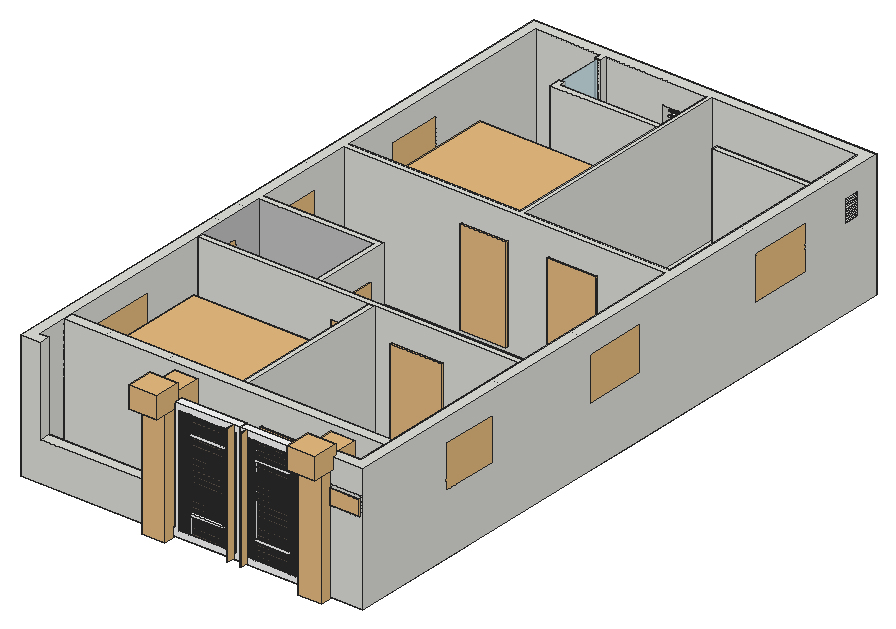
# SketchUp Ruby script. Lengths in inches.
U = 1.inch
M = Sketchup.active_model
def pt(a) = Geom::Point3d.new(a.map { |v| v * U })
def face(e, loops, mat)
  f = e.add_face(loops[0].map { |a| pt(a) })
  loops[1..].each { |l| e.add_face(l.map { |a| pt(a) }).erase! }
  f.material = f.back_material = mat if mat
  f
end
# faces: each face lists its corners as indices into pts; further lists are holes
def faces(e, pts, list, mat = nil) = list.each { |f| face(e, (f[0].is_a?(Array) ? f : [f]).map { |l| l.map { |i| pts[i] } }, mat) }
# xy, xz, yz: faces in a plane at the given z, y or x. An outline is a flat list of corners, or four numbers for a rectangle; further outlines are holes
def ring(l) = l.size == 4 ? [[l[0], l[1]], [l[2], l[1]], [l[2], l[3]], [l[0], l[3]]] : l.each_slice(2).to_a
def flat(e, list, mat, &to3) = list.each { |f| face(e, (f[0].is_a?(Array) ? f : [f]).map { |l| ring(l).map { |u, v| to3.(u, v) } }, mat) }
def xy(e, z, list, mat = nil) = flat(e, list, mat) { |x, y| [x, y, z] }
def xz(e, y, list, mat = nil) = flat(e, list, mat) { |x, z| [x, y, z] }
def yz(e, x, list, mat = nil) = flat(e, list, mat) { |y, z| [x, y, z] }
def lines(e, pts, list) = list.each { |a, b| e.add_line(pt(pts[a]), pt(pts[b])) }
# prism: a flat outline (further loops are holes) pulled along v
def prism(e, loops, v, mat = nil)
  f = face(e, loops, mat); d = Geom::Vector3d.new(v.map { |x| x * U })
  f.pushpull(f.normal.samedirection?(d) ? d.length : -d.length)
end
def box(e, o, s, mat = nil) = prism(e, [[o, [o[0] + s[0], o[1], o[2]], [o[0] + s[0], o[1] + s[1], o[2]], [o[0], o[1] + s[1], o[2]]]], [0, 0, s[2]], mat)
def at(x, y, z, deg = 0) = Geom::Transformation.translation(pt([x, y, z])) * Geom::Transformation.rotation(ORIGIN, Z_AXIS, deg.degrees)
def axes(o, x, y, z) = Geom::Transformation.new([*x, 0, *y, 0, *z, 0, *pt(o).to_a, 1])
def part(name) = M.definitions.add(name)
# library, detail: a bought-in or finely detailed component or shape, given as its bounding box
def library(name, o, s) = part(name).tap { |d| box(d.entities, o, s) }
def detail(e, o, s) = box(e.add_group.entities, o, s)
def put(e, d, t, mat = nil) = e.add_instance(d, t).tap { |i| i.material = mat if mat }
def group(e, t, mat = nil) = e.add_group.tap { |g| g.transformation = t; g.material = mat if mat }.entities
root = M.entities
M.materials.add("34af249def0fa13af67ab2bd33b938c5").color = [198, 197, 197]
M.materials.add("Steve_Edges").color = [0, 0, 0]
M.materials.add("[Color A04]").color = [128, 123, 118]
M.materials.add("[Color_000]").color = [255, 255, 255]
M.materials.add("[Color_C20]").color = [102, 91, 81]
M.materials.add("[Translucent Glass Safety]").color = [204, 235, 244]
M.materials["[Translucent Glass Safety]"].alpha = 0.5
c1 = library("A$C1EC128A1",[-3.37,-3.7,0],[6.74,7.4,0.01])
c2 = part("*U4")
p = [[-20,-17,0],[-20,23,0],[-18.25,23,0],[-18.25,-17,0],[20,-17,0],[19.92,-14.49,0],
  [19.68,-11.99,0],[19.29,-9.5,0],[18.74,-7.05,0],[18.04,-4.64,0],[17.19,-2.28,0],[16.19,0.03,0],
  [15.05,2.27,0],[13.77,4.43,0],[12.36,6.51,0],[10.82,8.5,0],[9.16,10.38,0],[7.38,12.16,0],
  [5.5,13.82,0],[3.51,15.36,0],[1.43,16.77,0],[-0.73,18.05,0],[-2.97,19.19,0],[-5.28,20.19,0],
  [-7.64,21.04,0],[-10.05,21.74,0],[-12.5,22.29,0],[-14.99,22.68,0],[-17.49,22.92,0],[-20,-23,0],
  [20,-23,0]]
lines(c2.entities,p,[[0,1],[1,2],[2,3],[3,0],[4,5],[5,6],[6,7],[7,8],[8,9],[9,10],[10,11],[11,12],
  [12,13],[13,14],[14,15],[15,16],[16,17],[17,18],[18,19],[19,20],[20,21],[21,22],[22,23],[23,24],
  [24,25],[25,26],[26,27],[27,28],[28,1],[0,29],[4,30]])
c3 = library("Кровать",[-17.4,-26.33,0],[117.11,127.46,87.48])
c4 = library("Plante \#58",[-0.43,-1.58,0],[20.84,18.06,17.59])
c5 = library("Wall mounted toilet",[0,0,0],[28.35,19.69,42.125])
c6 = library("RAGHU HOUSE NO:2",[0.29,0,0],[30,12.43,1])
c7 = part("Group20\#1")
xy(c7.entities,0,[[51,0,51,82.47,60,82.47,60,9,155.48,9,155.48,33.6875,161.25,33.6875,161.25,0],[309.375,0,309.375,9,330,9,330,96.75,339,96.75,339,0],[60,34,94.95,43],[94.95,34,147.28,37],[147.28,34,330,43],
  [94.95,39.54,147.28,43],[330,96.75,333.05,145.46],[333.05,96.75,335.78,145.46],[330,145.46,339,228.43],[60,175,330,180],
  [51,201.63,53.96,226.12],[56.65,201.63,60,226.12],[51,226.12,60,273.45],[332.92,228.43,335.82,280.48],[51,273.45,53.82,296.92],
  [330,407.14,332.19,455.17],[335.62,407.14,339,455.17],[51,416.55,51,540,146.27,540,146.27,531,119,531,119,525.5625,114,525.5625,114,531,60,531,60,416.55],[114,478,114,487.41,116.04,487.41,116.04,525.5625,116.5,525.5625,116.5,487.41,119,487.41,119,483,204,483,204,478],[250.49,478,330,483],
  [330,491.8,333.45,519.52],[333.45,491.8,336.34,519.52],[330,519.52,330,531,169.99,531,169.99,540,339,540,339,519.52]])
xy(c7.entities,4,[[226.66,34,272.82,43],[171.75,175,200.82,180],[223.46,175,266.65,180],[156,203.83,161,228.59],[158.97,329,197.75,334],
  [231.92,329,272.96,334]])
xy(c7.entities,33.15,[[67.875,0,161.25,0,161.25,33.6875,155.48,33.6875,155.48,9,67.875,9]])
xy(c7.entities,51,[[51,67.95,60,121.625],[330,87.84,339,136.4],[51,191.41,60,215.55],[330,239.56,339,290.25],[51,257.89,60,297.67],
  [51,379.57,60,425.91],[330,412.9375,339,464.66]])
xy(c7.entities,67.875,[[166.625,531,185.79,540]])
xy(c7.entities,68.5625,[[330,507.05,339,520.18]])
xy(c7.entities,84,[[226.66,34,272.82,43],[171.75,175,200.82,180],[223.46,175,266.65,180],[156,203.83,161,228.59],[158.97,329,197.75,334],
  [231.92,329,272.96,334]])
xy(c7.entities,87,[[51,67.95,60,121.625],[330,87.84,339,136.4],[51,191.41,60,215.55],[330,239.56,339,290.25],[51,257.89,60,297.67],
  [51,379.57,60,425.91],[330,412.9375,339,464.66],[330,507.05,339,520.18],[166.625,531,185.79,540]])
xy(c7.entities,106.3,[[[51,0,67.875,0,67.875,9,60,9,60,240,156,240,156,180,161,180,161,245,60,245,60,329,330,329,330,9,309.375,9,309.375,0,339,0,339,540,51,540],[60,334,60,531,114,531,114,525.5625,119,525.5625,119,531,204,531,204,334],[208,334,330,531]],[60,34,330,43],[204,43,209,175],[60,175,330,180],[114,478,204,478,204,483,119,483,119,487.41,116.5,487.41,116.5,525.5625,116.04,525.5625,116.04,487.41,114,487.41],
  [250.49,478,330,483]])
xz(c7.entities,0,[[51,0,161.25,0,161.25,33.15,67.875,33.15,67.875,106.3,51,106.3],[[309.375,0,339,106.3],[311.76,69.02,337.14,85.58]],[311.76,69.02,337.14,85.58]])
xz(c7.entities,9,[[60,0,60,106.3,67.875,106.3,67.875,33.15,155.48,33.15,155.48,0],[309.375,0,330,106.3]])
xz(c7.entities,33.6875,[[155.48,0,161.25,33.15]])
xz(c7.entities,34,[[[60,0,330,106.3],[226.66,4,272.82,84]]])
xz(c7.entities,43,[[60,0,204,106.3],[204,0,209,106.3],[[209,0,330,106.3],[226.66,4,272.82,84]]])
xz(c7.entities,67.95,[[51,51,60,87]])
xz(c7.entities,87.84,[[330,51,339,87]])
xz(c7.entities,121.625,[[51,51,60,87]])
xz(c7.entities,136.4,[[330,51,339,87]])
xz(c7.entities,175,[[[60,0,204,106.3],[171.75,4,200.82,84]],[204,0,209,106.3],[[209,0,330,106.3],[223.46,4,266.65,84]]])
xz(c7.entities,180,[[156,0,161,106.3],[[161,0,330,106.3],[223.46,4,266.65,84],[171.75,4,200.82,84]]])
xz(c7.entities,180,[[60,0,156,106.3]],"34af249def0fa13af67ab2bd33b938c5")
xz(c7.entities,191.41,[[51,51,60,87]])
xz(c7.entities,203.83,[[156,4,161,84]])
xz(c7.entities,215.55,[[51,51,60,87]])
xz(c7.entities,228.59,[[156,4,161,84]])
xz(c7.entities,239.56,[[330,51,339,87]])
xz(c7.entities,240,[[60,0,156,106.3]],"34af249def0fa13af67ab2bd33b938c5")
xz(c7.entities,245,[[60,0,161,106.3]])
xz(c7.entities,257.89,[[51,51,60,87]])
xz(c7.entities,290.25,[[330,51,339,87]])
xz(c7.entities,297.67,[[51,51,60,87]])
xz(c7.entities,329,[[[60,0,330,106.3],[231.92,4,272.96,84],[158.97,4,197.75,84]]])
xz(c7.entities,334,[[[60,0,204,106.3],[158.97,4,197.75,84]],[[208,0,330,106.3],[231.92,4,272.96,84]]])
xz(c7.entities,379.57,[[51,51,60,87]])
xz(c7.entities,412.9375,[[330,51,339,87]])
xz(c7.entities,425.91,[[51,51,60,87]])
xz(c7.entities,464.66,[[330,51,339,87]])
xz(c7.entities,478,[[114,0,204,106.3],[250.49,0,330,106.3]])
xz(c7.entities,483,[[119,0,204,106.3],[250.49,0,330,106.3]])
xz(c7.entities,487.41,[[114,0,116.04,106.3],[116.5,0,119,106.3]])
xz(c7.entities,507.05,[[330,68.5625,339,87]])
xz(c7.entities,520.18,[[330,68.5625,339,87]])
xz(c7.entities,525.5625,[[114,0,116.04,106.3],[116.5,0,119,106.3]])
xz(c7.entities,531,[[60,0,114,106.3],[[119,0,204,106.3],[166.625,67.875,185.79,87]],[208,0,330,106.3]])
xz(c7.entities,540,[[[51,0,339,106.3],[166.625,67.875,185.79,87]]])
yz(c7.entities,51,[[[0,0,540,106.3],[67.95,51,121.625,87],[379.57,51,425.91,87],[257.89,51,297.67,87],[191.41,51,215.55,87]]])
yz(c7.entities,60,[[9,0,34,106.3],[34,0,43,106.3],[[43,0,175,106.3],[67.95,51,121.625,87]],[175,0,180,106.3],[[245,0,329,106.3],[257.89,51,297.67,87]],
  [[334,0,531,106.3],[379.57,51,425.91,87]]])
yz(c7.entities,60,[[[180,0,240,106.3],[191.41,51,215.55,87]]],"34af249def0fa13af67ab2bd33b938c5")
yz(c7.entities,67.875,[[0,33.15,9,106.3]])
yz(c7.entities,114,[[478,0,487.41,106.3],[525.5625,0,531,106.3]])
yz(c7.entities,119,[[483,0,487.41,106.3],[525.5625,0,531,106.3]])
yz(c7.entities,155.48,[[9,0,33.6875,33.15]])
yz(c7.entities,156,[[[180,0,240,106.3],[203.83,4,228.59,84]]],"34af249def0fa13af67ab2bd33b938c5")
yz(c7.entities,158.97,[[329,4,334,84]])
yz(c7.entities,161,[[[180,0,245,106.3],[203.83,4,228.59,84]]])
yz(c7.entities,161.25,[[0,0,33.6875,33.15]])
yz(c7.entities,166.625,[[531,67.875,540,87]])
yz(c7.entities,171.75,[[175,4,180,84]])
yz(c7.entities,185.79,[[531,67.875,540,87]])
yz(c7.entities,197.75,[[329,4,334,84]])
yz(c7.entities,200.82,[[175,4,180,84]])
yz(c7.entities,204,[[43,0,175,106.3],[334,0,478,106.3],[478,0,483,106.3],[483,0,531,106.3]])
yz(c7.entities,208,[[334,0,531,106.3]])
yz(c7.entities,209,[[43,0,175,106.3]])
yz(c7.entities,223.46,[[175,4,180,84]])
yz(c7.entities,226.66,[[34,4,43,84]])
yz(c7.entities,231.92,[[329,4,334,84]])
yz(c7.entities,250.49,[[478,0,483,106.3]])
yz(c7.entities,266.65,[[175,4,180,84]])
yz(c7.entities,272.82,[[34,4,43,84]])
yz(c7.entities,272.96,[[329,4,334,84]])
yz(c7.entities,309.375,[[0,0,9,106.3]])
yz(c7.entities,330,[[9,0,34,106.3],[34,0,43,106.3],[[43,0,175,106.3],[87.84,51,136.4,87]],[175,0,180,106.3],[[180,0,329,106.3],[239.56,51,290.25,87]],
  [[334,0,478,106.3],[412.9375,51,464.66,87]],[478,0,483,106.3],[[483,0,531,106.3],[507.05,68.5625,520.18,87]]])
yz(c7.entities,339,[[[0,0,540,106.3],[412.9375,51,464.66,87],[239.56,51,290.25,87],[87.84,51,136.4,87],[507.05,68.5625,520.18,87]]])
p = [[94.95,39.54,0],[94.95,39.54,106.3],[335.78,145.46,0],[335.78,145.46,106.3],[335.82,228.43,0],[335.82,228.43,106.3],
  [336.34,491.8,0],[336.34,491.8,106.3],[332.19,407.14,0],[332.19,407.14,106.3],[94.95,37,0],[94.95,37,106.3],
  [333.45,491.8,0],[333.45,491.8,106.3],[53.82,296.92,0],[53.82,296.92,106.3],[147.28,39.54,0],[147.28,39.54,106.3],
  [53.96,226.12,0],[53.96,226.12,106.3],[147.28,37,0],[147.28,37,106.3],[335.62,407.14,0],[335.62,407.14,106.3],
  [53.96,201.63,0],[53.96,201.63,106.3],[333.05,145.46,0],[333.05,145.46,106.3],[332.92,228.43,0],[332.92,228.43,106.3],
  [56.65,226.12,0],[56.65,226.12,106.3],[56.65,201.63,0],[56.65,201.63,106.3]]
lines(c7.entities,p,[[0,1],[2,3],[4,5],[6,7],[8,9],[10,11],[12,13],[14,15],[16,17],[18,19],[20,21],[22,23],
  [24,25],[26,27],[28,29],[30,31],[32,33]])
put(c7.entities,c6,axes([311.98,0,70.4],[0.82,0,0],[0,0,1],[0,-1,0]),"Steve_Edges")
g1 = group(c7.entities,at(116.04,487.41,0),"[Translucent Glass Safety]")
yz(g1,0,[[0,0,38.16,106.3]])
yz(g1,0.46,[[0,0,38.16,106.3]])
c8 = library("Group\#2",[0,0,0],[9.07,48.5625,36])
c9 = library("Group\#4",[0,0,0],[9.07,50.69,36])
c10 = library("Group\#6",[0,0,0],[9.07,51.72,36])
c11 = library("Group\#12",[0,0,0],[9.07,46.34,36])
c12 = library("Group\#14",[0,0,0],[9.07,39.78,36])
c13 = library("Group\#16",[0,0,0],[9.07,24.15,36])
c14 = library("Group\#18",[0,0,0],[9.07,53.68,36])
c15 = part("Group44\#1")
p = [[-6.5625,-7.63,1.2],[6.5625,-7.63,1.2],[6.5625,-7.75,0.39],[-6.5625,-7.75,0.39],[-6.5625,-7.67,2.01],[6.5625,-7.67,2.01],
  [-6.5625,-7.85,2.79],[6.5625,-7.85,2.79],[-6.5625,-8.19,3.53],[6.5625,-8.19,3.53],[-6.5625,-8.66,4.19],[6.5625,-8.66,4.19],
  [-6.5625,-9.22,4.72],[6.5625,-9.22,4.72]]
faces(c15.entities,p,[[0,1,2,3],[4,5,1,0],[6,7,5,4],[8,9,7,6],[10,11,9,8],[11,10,12,13]])
c16 = part("Group45\#1")
p = [[-6.5625,-3.69,1.2],[6.5625,-3.69,1.2],[6.5625,-3.8125,0.39],[-6.5625,-3.8125,0.39],[-6.5625,-3.73,2.01],[6.5625,-3.73,2.01],
  [-6.5625,-3.92,2.79],[6.5625,-3.92,2.79],[-6.5625,-4.25,3.53],[6.5625,-4.25,3.53],[-6.5625,-4.72,4.19],[6.5625,-4.72,4.19],
  [-6.5625,-5.3125,4.75],[6.5625,-5.3125,4.75],[-6.5625,-6,5.18],[6.5625,-6,5.18],[-6.5625,-6.75,5.48],[6.5625,-6.75,5.48]]
faces(c16.entities,p,[[0,1,2,3],[4,5,1,0],[6,7,5,4],[8,9,7,6],[10,11,9,8],[12,13,11,10],[14,15,13,12],[16,17,15,14]])
c17 = part("Group46\#1")
p = [[6.5625,0.125,0.39],[-6.5625,0.125,0.39],[-6.5625,0.25,1.2],[6.5625,0.25,1.2],[-6.5625,0.21,2.01],[6.5625,0.21,2.01],
  [-6.5625,0.02,2.79],[6.5625,0.02,2.79],[-6.5625,-0.32,3.53],[6.5625,-0.32,3.53],[-6.5625,-0.79,4.19],[6.5625,-0.79,4.19],
  [-6.5625,-1.375,4.75],[6.5625,-1.375,4.75],[-6.5625,-2.06,5.18],[6.5625,-2.06,5.18],[-6.5625,-2.8125,5.48],[6.5625,-2.8125,5.48]]
faces(c17.entities,p,[[0,1,2,3],[3,2,4,5],[5,4,6,7],[7,6,8,9],[9,8,10,11],[11,10,12,13],[13,12,14,15],[15,14,16,17]])
c18 = part("Group47\#1")
p = [[6.5625,4.0625,0.39],[-6.5625,4.0625,0.39],[-6.5625,4.18,1.2],[6.5625,4.18,1.2],[-6.5625,4.15,2.01],[6.5625,4.15,2.01],
  [-6.5625,3.96,2.79],[6.5625,3.96,2.79],[-6.5625,3.62,3.53],[6.5625,3.62,3.53],[-6.5625,3.15,4.19],[6.5625,3.15,4.19],
  [-6.5625,2.5625,4.75],[6.5625,2.5625,4.75],[-6.5625,1.88,5.18],[6.5625,1.88,5.18],[-6.5625,1.125,5.48],[6.5625,1.125,5.48]]
faces(c18.entities,p,[[0,1,2,3],[3,2,4,5],[5,4,6,7],[7,6,8,9],[9,8,10,11],[11,10,12,13],[13,12,14,15],[15,14,16,17]])
c19 = part("Group48\#1")
p = [[6.5625,8,0.39],[-6.5625,8,0.39],[-6.5625,8.12,1.2],[6.5625,8.12,1.2],[-6.5625,8.08,2.01],[6.5625,8.08,2.01],
  [-6.5625,7.9,2.79],[6.5625,7.9,2.79],[-6.5625,7.56,3.53],[6.5625,7.56,3.53],[-6.5625,7.09,4.19],[6.5625,7.09,4.19],
  [-6.5625,6.5,4.75],[6.5625,6.5,4.75],[-6.5625,5.82,5.18],[6.5625,5.82,5.18],[-6.5625,5.0625,5.48],[6.5625,5.0625,5.48]]
faces(c19.entities,p,[[0,1,2,3],[3,2,4,5],[5,4,6,7],[7,6,8,9],[9,8,10,11],[11,10,12,13],[13,12,14,15],[15,14,16,17]])
c20 = part("Group42\#1")
put(c20.entities,c15,at(0,0,0))
put(c20.entities,c16,at(0,0,0))
put(c20.entities,c17,at(0,0,0))
put(c20.entities,c18,at(0,0,0))
put(c20.entities,c19,at(0,0,0))
c21 = part("Group50\#1")
p = [[-9.58,-7.97,1.2],[9.58,-7.97,1.2],[9.58,-8.09,0.39],[-9.58,-8.09,0.39],[-9.58,-8.01,2.01],[9.58,-8.01,2.01],
  [-9.58,-8.2,2.79],[9.58,-8.2,2.79],[-9.58,-8.53,3.53],[9.58,-8.53,3.53],[-9.58,-9,4.19],[9.58,-9,4.19],
  [-9.58,-9.5625,4.72],[9.58,-9.5625,4.72]]
faces(c21.entities,p,[[0,1,2,3],[4,5,1,0],[6,7,5,4],[8,9,7,6],[10,11,9,8],[11,10,12,13]])
c22 = part("Group51\#1")
p = [[-9.58,-4.04,1.2],[9.58,-4.04,1.2],[9.58,-4.16,0.39],[-9.58,-4.16,0.39],[-9.58,-4.07,2.01],[9.58,-4.07,2.01],
  [-9.58,-4.26,2.79],[9.58,-4.26,2.79],[-9.58,-4.6,3.53],[9.58,-4.6,3.53],[-9.58,-5.07,4.19],[9.58,-5.07,4.19],
  [-9.58,-5.66,4.75],[9.58,-5.66,4.75],[-9.58,-6.34,5.18],[9.58,-6.34,5.18],[-9.58,-7.09,5.48],[9.58,-7.09,5.48]]
faces(c22.entities,p,[[0,1,2,3],[4,5,1,0],[6,7,5,4],[8,9,7,6],[10,11,9,8],[12,13,11,10],[14,15,13,12],[16,17,15,14]])
c23 = part("Group52\#1")
p = [[-9.58,-0.1,1.2],[9.58,-0.1,1.2],[9.58,-0.22,0.39],[-9.58,-0.22,0.39],[-9.58,-0.13,2.01],[9.58,-0.13,2.01],
  [-9.58,-0.32,2.79],[9.58,-0.32,2.79],[-9.58,-0.66,3.53],[9.58,-0.66,3.53],[-9.58,-1.13,4.19],[9.58,-1.13,4.19],
  [-9.58,-1.72,4.75],[9.58,-1.72,4.75],[-9.58,-2.4,5.18],[9.58,-2.4,5.18],[-9.58,-3.16,5.48],[9.58,-3.16,5.48]]
faces(c23.entities,p,[[0,1,2,3],[4,5,1,0],[6,7,5,4],[8,9,7,6],[10,11,9,8],[12,13,11,10],[14,15,13,12],[16,17,15,14]])
c24 = part("Group53\#1")
p = [[-9.58,3.84,1.2],[9.58,3.84,1.2],[9.58,3.72,0.39],[-9.58,3.72,0.39],[-9.58,3.8,2.01],[9.58,3.8,2.01],
  [-9.58,3.61,2.79],[9.58,3.61,2.79],[-9.58,3.28,3.53],[9.58,3.28,3.53],[-9.58,2.81,4.19],[9.58,2.81,4.19],
  [-9.58,2.22,4.75],[9.58,2.22,4.75],[-9.58,1.54,5.18],[9.58,1.54,5.18],[-9.58,0.78,5.48],[9.58,0.78,5.48]]
faces(c24.entities,p,[[0,1,2,3],[4,5,1,0],[6,7,5,4],[8,9,7,6],[10,11,9,8],[12,13,11,10],[14,15,13,12],[16,17,15,14]])
c25 = part("Group54\#1")
p = [[-9.58,7.78,1.2],[9.58,7.78,1.2],[9.58,7.66,0.39],[-9.58,7.66,0.39],[-9.58,7.74,2.01],[9.58,7.74,2.01],
  [-9.58,7.55,2.79],[9.58,7.55,2.79],[-9.58,7.22,3.53],[9.58,7.22,3.53],[-9.58,6.75,4.19],[9.58,6.75,4.19],
  [-9.58,6.16,4.75],[9.58,6.16,4.75],[-9.58,5.47,5.18],[9.58,5.47,5.18],[-9.58,4.72,5.48],[9.58,4.72,5.48]]
faces(c25.entities,p,[[0,1,2,3],[4,5,1,0],[6,7,5,4],[8,9,7,6],[10,11,9,8],[12,13,11,10],[14,15,13,12],[16,17,15,14]])
c26 = part("Group48\#2")
put(c26.entities,c21,at(0,0,0))
put(c26.entities,c22,at(0,0,0))
put(c26.entities,c23,at(0,0,0))
put(c26.entities,c24,at(0,0,0))
put(c26.entities,c25,at(0,0,0))
c27 = library("Group\#7",[0,0,0],[46.15,10.47,80])
c28 = library("Group\#8",[0,0,0],[43.18,6.6,80])
c29 = library("Group\#9",[0,0,0],[29.0625,6.6,80])
c30 = library("Group\#10",[0,0,0],[6.6,24.76,80])
c31 = library("Group\#19",[0,0,0],[41.04,6.6,80])
c32 = library("Gate post",[0,0,0],[97.06,71.13,326.45])
c33 = part("Horizontal gate slat")
xy(c33.entities,0,[[0.39,114.16,6.3,114.17]])
xy(c33.entities,0,[[0.39,0,6.3,114.16]],"[Color_C20]")
xy(c33.entities,0.39,[[0.39,0,0.79,114.17],[0.98,0,2.07,114.17],[2.36,0,3.2,114.17],[3.59,0,4.37,114.17],[4.56,0,5.71,114.17],
  [5.91,0,6.3,114.17]],"[Color_C20]")
xy(c33.entities,0.79,[[0.39,0,0.79,114.17],[0.98,0,2.07,114.17],[2.36,0,3.2,114.17],[3.59,0,4.37,114.17],[4.56,0,5.71,114.17],
  [5.91,0,6.3,114.17]],"[Color_C20]")
xy(c33.entities,0.99,[[1.13,0,1.21,114.16],[1.87,0,1.94,114.16],[2.61,0,2.68,114.16],[3.35,0,3.42,114.16],[4.08,0,4.16,114.16],
  [4.82,0,4.9,114.16],[5.5625,0,5.63,114.16],[6.3,0,6.37,114.16]],"[Color_C20]")
xy(c33.entities,1.18,[[0.39,114.16,3.35,114.17],[3.35,114.16,6.3,114.17]])
xy(c33.entities,1.18,[[0.39,0,1.13,114.16],[1.21,0,1.87,114.16],[1.94,0,2.61,114.16],[2.68,0,3.35,114.16],[3.42,0,4.08,114.16],
  [4.16,0,4.82,114.16],[4.9,0,5.5625,114.16],[5.63,0,6.3,114.16]],"[Color_C20]")
xz(c33.entities,0,[[[0.39,0,6.3,0,6.3,0.39,5.91,0.39,5.91,0.79,6.3,0.79,6.3,1.18,5.63,1.18,5.63,0.99,5.5625,0.99,5.5625,1.18,4.9,1.18,4.9,0.99,4.82,0.99,4.82,1.18,4.16,1.18,4.16,0.99,4.08,0.99,4.08,1.18,3.42,1.18,3.42,0.99,3.35,0.99,3.35,1.18,2.68,1.18,2.68,0.99,2.61,0.99,2.61,1.18,1.94,1.18,1.94,0.99,1.87,0.99,1.87,1.18,1.21,1.18,1.21,0.99,1.13,0.99,1.13,1.18,0.39,1.18,0.39,0.79,0.79,0.79,0.79,0.39,0.39,0.39],[4.56,0.39,5.71,0.79],[0.98,0.39,2.07,0.79],[2.36,0.39,3.2,0.79],[3.59,0.39,4.37,0.79]],[6.3,0.99,6.37,1.18]],"[Color_C20]")
xz(c33.entities,114.16,[[1.13,0.99,1.21,1.18],[1.87,0.99,1.94,1.18],[2.61,0.99,2.68,1.18],[3.35,0.99,3.42,1.18],[4.08,0.99,4.16,1.18],
  [4.82,0.99,4.9,1.18],[5.5625,0.99,5.63,1.18]],"[Color_C20]")
xz(c33.entities,114.17,[[[0.39,0,0.39,0.39,0.79,0.39,0.79,0.79,0.39,0.79,0.39,1.18,6.3,1.18,6.3,0.79,5.91,0.79,5.91,0.39,6.3,0.39,6.3,0],[4.56,0.39,5.71,0.79],[0.98,0.39,2.07,0.79],[2.36,0.39,3.2,0.79],[3.59,0.39,4.37,0.79]]],"[Color_C20]")
yz(c33.entities,0.39,[[114.16,0,114.17,0.39],[114.16,0.79,114.17,1.18]])
yz(c33.entities,0.39,[[0,0,114.16,0.39],[0,0.79,114.16,1.18]],"[Color_C20]")
yz(c33.entities,0.79,[[0,0.39,114.17,0.79]],"[Color_C20]")
yz(c33.entities,0.98,[[0,0.39,114.17,0.79]],"[Color_C20]")
yz(c33.entities,1.13,[[0,0.99,114.16,1.18]],"[Color_C20]")
yz(c33.entities,1.21,[[0,0.99,114.16,1.18]],"[Color_C20]")
yz(c33.entities,1.87,[[0,0.99,114.16,1.18]],"[Color_C20]")
yz(c33.entities,1.94,[[0,0.99,114.16,1.18]],"[Color_C20]")
yz(c33.entities,2.07,[[0,0.39,114.17,0.79]],"[Color_C20]")
yz(c33.entities,2.36,[[0,0.39,114.17,0.79]],"[Color_C20]")
yz(c33.entities,2.61,[[0,0.99,114.16,1.18]],"[Color_C20]")
yz(c33.entities,2.68,[[0,0.99,114.16,1.18]],"[Color_C20]")
yz(c33.entities,3.2,[[0,0.39,114.17,0.79]],"[Color_C20]")
yz(c33.entities,3.35,[[0,0.99,114.16,1.18]],"[Color_C20]")
yz(c33.entities,3.42,[[0,0.99,114.16,1.18]],"[Color_C20]")
yz(c33.entities,3.59,[[0,0.39,114.17,0.79]],"[Color_C20]")
yz(c33.entities,4.08,[[0,0.99,114.16,1.18]],"[Color_C20]")
yz(c33.entities,4.16,[[0,0.99,114.16,1.18]],"[Color_C20]")
yz(c33.entities,4.37,[[0,0.39,114.17,0.79]],"[Color_C20]")
yz(c33.entities,4.56,[[0,0.39,114.17,0.79]],"[Color_C20]")
yz(c33.entities,4.82,[[0,0.99,114.16,1.18]],"[Color_C20]")
yz(c33.entities,4.9,[[0,0.99,114.16,1.18]],"[Color_C20]")
yz(c33.entities,5.5625,[[0,0.99,114.16,1.18]],"[Color_C20]")
yz(c33.entities,5.63,[[0,0.99,114.16,1.18]],"[Color_C20]")
yz(c33.entities,5.71,[[0,0.39,114.17,0.79]],"[Color_C20]")
yz(c33.entities,5.91,[[0,0.39,114.17,0.79]],"[Color_C20]")
yz(c33.entities,6.3,[[114.16,0,114.17,0.39],[114.16,0.79,114.17,1.18]])
yz(c33.entities,6.3,[[0,0,114.16,0.39],[0,0.79,114.16,0.99],[0,0.99,114.16,1.18]],"[Color_C20]")
yz(c33.entities,6.37,[[0,0.99,114.16,1.18]],"[Color_C20]")
p = [[0,0,0],[0.39,0,0]]
lines(c33.entities,p,[[0,1]])
c34 = part("Vertical gate panel")
put(c34.entities,c33,axes([0,1.18,0],[3.67755,0,0],[0,0,2.40086],[0,-1,0]))
put(c34.entities,c33,axes([21.72,1.18,0],[3.67755,0,0],[0,0,2.40086],[0,-1,0]))
c35 = library("Gate pull handle",[-0.01,0,0],[1.26,2.875,48])
c36 = part("Double entrance gate")
xy(c36.entities,0,[[553.15,18.86,552.64,18.92,552.18,19.1,551.78,19.39,551.47,19.76,551.27,20.2,551.21,20.67,551.27,21.13,551.47,21.57,551.78,21.94,552.18,22.23,552.64,22.41,553.15,22.47,553.65,22.41,554.11,22.23,554.52,21.94,554.82,21.57,555.02,21.13,555.08,20.67,555.02,20.2,554.82,19.76,554.52,19.39,554.11,19.1,553.65,18.92],[12.73,19.29,12.23,19.35,11.76,19.55,11.36,19.85,11.05,20.25,10.86,20.72,10.79,21.22,10.86,21.72,11.05,22.19,11.36,22.59,11.76,22.9,12.23,23.09,12.73,23.16,13.23,23.09,13.7,22.9,14.1,22.59,14.41,22.19,14.6,21.72,14.67,21.22,14.6,20.72,14.41,20.25,14.1,19.85,13.7,19.55,13.23,19.35]])
xy(c36.entities,5.93,[[[4.54,12.88,282.375,27.63],[12.73,19.29,13.23,19.35,13.7,19.55,14.1,19.85,14.41,20.25,14.6,20.72,14.67,21.22,14.6,21.72,14.41,22.19,14.1,22.59,13.7,22.9,13.23,23.09,12.73,23.16,12.23,23.09,11.76,22.9,11.36,22.59,11.05,22.19,10.86,21.72,10.79,21.22,10.86,20.72,11.05,20.25,11.36,19.85,11.76,19.55,12.23,19.35]],[[283.5,12.88,556.09,26.65],[553.15,18.86,553.65,18.92,554.11,19.1,554.52,19.39,554.82,19.76,555.02,20.2,555.08,20.67,555.02,21.13,554.82,21.57,554.52,21.94,554.11,22.23,553.65,22.41,553.15,22.47,552.64,22.41,552.18,22.23,551.78,21.94,551.47,21.57,551.27,21.13,551.21,20.67,551.27,20.2,551.47,19.76,551.78,19.39,552.18,19.1,552.64,18.92]]],"[Color_000]")
xy(c36.entities,21.29,[[73.46,12.88,80.01,15.32],[80.01,12.88,217.27,15.32],[217.27,12.88,223.83,15.32],[342.04,12.88,348.6,15.16],[348.6,12.88,485.86,15.16],
  [485.86,12.88,492.42,15.16]])
xy(c36.entities,21.29,[[30.27,12.88,51.87,27.63],[51.87,12.88,73.46,27.63],[223.83,12.88,267.01,15.32],[298.86,12.88,342.04,15.16],[492.42,12.88,514.01,26.65],
  [514.01,12.88,535.6,26.65],[298.86,15.16,342.04,26.65],[348.6,15.16,485.86,26.65],[80.01,15.32,217.27,27.63],[223.83,15.32,267.01,27.63]],"[Color_000]")
xy(c36.entities,27.1,[[4.54,12.88,14.91,27.63],[550.96,12.88,556.09,26.65]],"[Color_000]")
xy(c36.entities,64.47,[[80.01,12.88,217.27,27.63],[348.6,12.88,485.86,26.65]],"[Color_000]")
xy(c36.entities,71.03,[[80.01,12.88,217.27,27.63],[348.6,12.88,485.86,26.65]],"[Color_000]")
xy(c36.entities,245.66,[[80.01,12.88,217.27,27.63],[348.6,12.88,485.86,26.65]],"[Color_000]")
xy(c36.entities,252.22,[[80.01,12.88,217.27,27.63],[348.6,12.88,485.86,26.65]],"[Color_000]")
xy(c36.entities,253.46,[[550.96,17.74,555.84,22.93],[10.04,18.09,14.91,23.65]],"[Color_000]")
xy(c36.entities,263.88,[[550.96,17.74,555.84,22.93],[10.04,18.09,14.91,23.65]],"[Color_000]")
xy(c36.entities,264.34,[[550.96,17.74,555.84,22.93],[555.84,17.74,565.875,22.93],[0,18.09,10.04,23.65],[10.04,18.09,14.91,23.65]],"[Color_000]")
xy(c36.entities,267.5,[[550.96,17.74,555.84,22.93],[555.84,17.74,565.875,22.93],[0,18.09,10.04,23.65],[10.04,18.09,14.91,23.65]],"[Color_000]")
xy(c36.entities,268.01,[[550.96,17.74,555.84,22.93],[10.04,18.09,14.91,23.65]],"[Color_000]")
xy(c36.entities,278.02,[[550.96,17.74,555.84,22.93],[10.04,18.09,14.91,23.65]],"[Color_000]")
xy(c36.entities,295.4,[[30.27,12.88,51.87,27.63],[51.87,12.88,73.46,27.63],[80.01,12.88,217.27,27.63],[223.83,12.88,267.01,27.63],[298.86,12.88,342.04,26.65],
  [348.6,12.88,485.86,26.65],[492.42,12.88,514.01,26.65],[514.01,12.88,535.6,26.65]],"[Color_000]")
xy(c36.entities,310.76,[[14.91,12.88,282.375,27.63],[283.5,12.88,550.96,26.65]],"[Color_000]")
xz(c36.entities,12.88,[[[4.54,5.93,282.375,5.93,282.375,310.76,14.91,310.76,14.91,27.1,4.54,27.1],[30.27,21.29,267.01,295.4]],[[283.5,5.93,556.09,5.93,556.09,27.1,550.96,27.1,550.96,310.76,283.5,310.76],[298.86,21.29,535.6,295.4]],[73.46,21.29,80.01,64.47],[217.27,21.29,223.83,64.47],[342.04,21.29,348.6,64.47],
  [485.86,21.29,492.42,64.47],[73.46,64.47,223.83,64.47,223.83,252.22,73.46,252.22,73.46,245.66,217.27,245.66,217.27,71.03,80.01,71.03,80.01,245.66,73.46,245.66],[342.04,64.47,492.42,64.47,492.42,245.66,485.86,245.66,485.86,71.03,348.6,71.03,348.6,245.66,492.42,245.66,492.42,252.22,342.04,252.22],[73.46,252.22,80.01,295.4],[217.27,252.22,223.83,295.4],
  [342.04,252.22,348.6,295.4],[485.86,252.22,492.42,295.4]],"[Color_000]")
xz(c36.entities,17.74,[[550.96,253.46,555.84,263.88],[550.96,264.34,565.875,267.5],[550.96,268.01,555.84,278.02]],"[Color_000]")
xz(c36.entities,18.09,[[10.04,253.46,14.91,263.88],[0,264.34,14.91,267.5],[10.04,268.01,14.91,278.02]],"[Color_000]")
xz(c36.entities,22.93,[[550.96,253.46,555.84,263.88],[550.96,264.34,555.84,265.59],[555.84,264.34,555.84,265.59,550.96,265.59,550.96,267.5,565.875,267.5,565.875,264.34],[550.96,268.01,555.84,278.02]],"[Color_000]")
xz(c36.entities,23.65,[[10.04,253.46,14.91,263.88],[0,264.34,0,267.5,14.91,267.5,14.91,265.59,10.04,265.59,10.04,264.34],[10.04,264.34,14.91,265.59],[10.04,268.01,14.91,278.02]],"[Color_000]")
xz(c36.entities,26.65,[[[283.5,5.93,283.5,310.76,550.96,310.76,550.96,27.1,556.09,27.1,556.09,5.93],[348.6,71.03,485.86,245.66],[492.42,21.29,535.6,295.4],[298.86,21.29,342.04,295.4],[348.6,252.22,485.86,295.4],[348.6,21.29,485.86,64.47]]],"[Color_000]")
xz(c36.entities,27.63,[[[4.54,5.93,4.54,27.1,14.91,27.1,14.91,310.76,282.375,310.76,282.375,5.93],[80.01,71.03,217.27,245.66],[30.27,21.29,73.46,295.4],[223.83,21.29,267.01,295.4],[80.01,252.22,217.27,295.4],[80.01,21.29,217.27,64.47]]],"[Color_000]")
yz(c36.entities,0,[[18.09,264.34,23.65,267.5]],"[Color_000]")
yz(c36.entities,4.54,[[12.88,5.93,27.63,27.1]],"[Color_000]")
yz(c36.entities,10.04,[[18.09,253.46,23.65,263.88],[18.09,268.01,23.65,278.02]],"[Color_000]")
yz(c36.entities,14.91,[[[12.88,27.1,27.63,310.76],[18.09,253.46,23.65,263.88],[18.09,268.01,23.65,278.02],[18.09,264.34,23.65,267.5]]],"[Color_000]")
yz(c36.entities,30.27,[[12.88,21.29,27.63,295.4]],"[Color_000]")
yz(c36.entities,73.46,[[12.88,21.29,27.63,64.47],[12.88,64.47,27.63,245.66],[12.88,245.66,27.63,252.22],[12.88,252.22,27.63,295.4]],"[Color_000]")
yz(c36.entities,80.01,[[12.88,21.29,27.63,64.47],[12.88,71.03,27.63,245.66],[12.88,252.22,27.63,295.4]],"[Color_000]")
yz(c36.entities,217.27,[[12.88,21.29,27.63,64.47],[12.88,71.03,27.63,245.66],[12.88,252.22,27.63,295.4]],"[Color_000]")
yz(c36.entities,223.83,[[12.88,21.29,27.63,64.47],[12.88,64.47,27.63,252.22],[12.88,252.22,27.63,295.4]],"[Color_000]")
yz(c36.entities,267.01,[[12.88,21.29,27.63,295.4]],"[Color_000]")
yz(c36.entities,282.375,[[12.88,5.93,27.63,310.76]],"[Color_000]")
yz(c36.entities,283.5,[[12.88,5.93,26.65,310.76]],"[Color_000]")
yz(c36.entities,298.86,[[12.88,21.29,26.65,295.4]],"[Color_000]")
yz(c36.entities,342.04,[[12.88,21.29,26.65,64.47],[12.88,64.47,26.65,252.22],[12.88,252.22,26.65,295.4]],"[Color_000]")
yz(c36.entities,348.6,[[12.88,21.29,26.65,64.47],[12.88,71.03,26.65,245.66],[12.88,252.22,26.65,295.4]],"[Color_000]")
yz(c36.entities,485.86,[[12.88,21.29,26.65,64.47],[12.88,71.03,26.65,245.66],[12.88,252.22,26.65,295.4]],"[Color_000]")
yz(c36.entities,492.42,[[12.88,21.29,26.65,64.47],[12.88,64.47,26.65,245.66],[12.88,245.66,26.65,252.22],[12.88,252.22,26.65,295.4]],"[Color_000]")
yz(c36.entities,535.6,[[12.88,21.29,26.65,295.4]],"[Color_000]")
yz(c36.entities,550.96,[[[12.88,27.1,26.65,310.76],[17.74,253.46,17.74,263.88,22.93,263.88,22.93,264.34,17.74,264.34,17.74,267.5,22.93,267.5,22.93,253.46],[17.74,268.01,22.93,278.02]]],"[Color_000]")
yz(c36.entities,555.84,[[17.74,253.46,22.93,263.88],[17.74,268.01,22.93,278.02]],"[Color_000]")
yz(c36.entities,556.09,[[12.88,5.93,26.65,27.1]],"[Color_000]")
p = [[552.64,18.92,5.93],[552.18,19.1,5.93],[552.18,19.1,0],[552.64,18.92,0],[553.15,18.86,5.93],[553.15,18.86,0],
  [553.65,18.92,5.93],[553.65,18.92,0],[554.11,19.1,5.93],[554.11,19.1,0],[551.78,19.39,5.93],[551.78,19.39,0],
  [554.52,19.39,5.93],[554.52,19.39,0],[12.73,19.29,5.93],[12.23,19.35,5.93],[12.23,19.35,0],[12.73,19.29,0],
  [13.23,19.35,5.93],[13.23,19.35,0],[11.76,19.55,5.93],[11.76,19.55,0],[13.7,19.55,5.93],[13.7,19.55,0],
  [551.47,19.76,5.93],[551.47,19.76,0],[554.82,19.76,5.93],[554.82,19.76,0],[11.36,19.85,5.93],[11.36,19.85,0],
  [14.1,19.85,5.93],[14.1,19.85,0],[551.27,20.2,5.93],[551.27,20.2,0],[555.02,20.2,5.93],[555.02,20.2,0],
  [11.05,20.25,5.93],[11.05,20.25,0],[14.41,20.25,5.93],[14.41,20.25,0],[551.21,20.67,5.93],[551.21,20.67,0],
  [555.08,20.67,5.93],[555.08,20.67,0],[10.86,20.72,5.93],[10.86,20.72,0],[14.6,20.72,5.93],[14.6,20.72,0],
  [10.79,21.22,5.93],[10.79,21.22,0],[14.67,21.22,5.93],[14.67,21.22,0],[551.27,21.13,5.93],[551.27,21.13,0],
  [555.02,21.13,5.93],[555.02,21.13,0],[551.47,21.57,5.93],[551.47,21.57,0],[554.82,21.57,5.93],[554.82,21.57,0],
  [10.86,21.72,5.93],[10.86,21.72,0],[14.6,21.72,5.93],[14.6,21.72,0],[551.78,21.94,5.93],[551.78,21.94,0],
  [554.52,21.94,5.93],[554.52,21.94,0],[11.05,22.19,5.93],[11.05,22.19,0],[14.41,22.19,5.93],[14.41,22.19,0],
  [552.18,22.23,5.93],[552.18,22.23,0],[554.11,22.23,5.93],[554.11,22.23,0],[11.36,22.59,5.93],[11.36,22.59,0],
  [14.1,22.59,5.93],[14.1,22.59,0],[552.64,22.41,5.93],[552.64,22.41,0],[553.65,22.41,5.93],[553.65,22.41,0],
  [553.15,22.47,5.93],[553.15,22.47,0],[11.76,22.9,5.93],[11.76,22.9,0],[13.7,22.9,5.93],[13.7,22.9,0],
  [12.23,23.09,5.93],[12.23,23.09,0],[13.23,23.09,5.93],[13.23,23.09,0],[12.73,23.16,5.93],[12.73,23.16,0],
  [495.13,15.16,21.29],[492.42,15.16,21.29],[505.99,15.16,295.37],[348.6,15.16,295.37],[485.84,15.16,253.84],[485.84,15.16,71.03],
  [59.88,15.32,295.37],[217.27,15.32,295.37],[70.74,15.32,21.29],[73.46,15.32,21.29],[80.03,15.32,253.84],[80.03,15.32,71.03],
  [282.375,12.88,5.93],[283.5,12.88,5.93],[14.91,23.65,264.34],[14.91,23.65,263.88]]
faces(c36.entities,p,[[0,1,2,3],[4,0,3,5],[6,4,5,7],[8,6,7,9],[1,10,11,2],[12,8,9,13],[14,15,16,17],[18,14,17,19],
  [15,20,21,16],[22,18,19,23],[10,24,25,11],[26,12,13,27],[20,28,29,21],[30,22,23,31],[24,32,33,25],[34,26,27,35],
  [28,36,37,29],[38,30,31,39],[32,40,41,33],[42,34,35,43],[36,44,45,37],[46,38,39,47],[44,48,49,45],[50,46,47,51],
  [40,52,53,41],[54,42,43,55],[52,56,57,53],[58,54,55,59],[48,60,61,49],[62,50,51,63],[56,64,65,57],[66,58,59,67],
  [60,68,69,61],[70,62,63,71],[64,72,73,65],[74,66,67,75],[68,76,77,69],[78,70,71,79],[72,80,81,73],[82,74,75,83],
  [80,84,85,81],[84,82,83,85],[76,86,87,77],[88,78,79,89],[86,90,91,87],[92,88,89,93],[90,94,95,91],[94,92,93,95]],"[Color_000]")
lines(c36.entities,p,[[96,97],[98,99],[100,101],[102,103],[104,105],[106,107],[108,109],[110,111]])
put(c36.entities,c34,axes([217.26,15.32,19.8125],[0,0,1.01983],[0,1,0],[-0.50074,0,0]))
put(c36.entities,c33,axes([222.13,16.5,21.29],[3.67755,0,0],[0,0,2.40086],[0,-1,0]))
put(c36.entities,c34,axes([217.29,15.32,113.92],[0,0,0.9999],[0,1,0],[-0.50074,0,0]))
put(c36.entities,c34,axes([217.27,15.32,200.78],[0,0,0.9999],[0,1,0],[-0.50074,0,0]))
put(c36.entities,c34,axes([217.29,15.32,70.49],[0,0,0.9999],[0,1,0],[-0.50074,0,0]))
put(c36.entities,c34,axes([217.27,15.32,249.59],[0,0,1.01983],[0,1,0],[-0.50074,0,0]))
put(c36.entities,c34,axes([217.27,15.32,157.35],[0,0,0.9999],[0,1,0],[-0.50074,0,0]))
put(c36.entities,c35,axes([253.77,0,7.15],[4.3,0,0],[0,4.47827,0],[0,0,6.3253]))
put(c36.entities,c33,axes([322.03,16.26,21.29],[-3.67755,0,0],[0,0,2.40086],[0,-0.93319,0]))
put(c36.entities,c33,axes([28.57,16.5,21.29],[3.67755,0,0],[0,0,2.40086],[0,-1,0]))
put(c36.entities,c33,axes([243.85,16.5,21.29],[3.67755,0,0],[0,0,2.40086],[0,-1,0]))
put(c36.entities,c33,axes([50.29,16.5,21.29],[3.67755,0,0],[0,0,2.40086],[0,-1,0]))
put(c36.entities,c34,axes([348.62,15.16,19.8125],[0,0,1.01983],[0,0.93319,0],[0.50074,0,0]))
put(c36.entities,c34,axes([348.6,15.16,249.59],[0,0,1.01983],[0,0.93319,0],[0.50074,0,0]))
put(c36.entities,c34,axes([348.6,15.16,200.78],[0,0,0.9999],[0,0.93319,0],[0.50074,0,0]))
put(c36.entities,c33,axes([537.3,16.26,21.29],[-3.67755,0,0],[0,0,2.40086],[0,-0.93319,0]))
put(c36.entities,c33,axes([515.58,16.26,21.29],[-3.67755,0,0],[0,0,2.40086],[0,-0.93319,0]))
put(c36.entities,c35,axes([312.11,0.86,7.15],[-4.3,0,0],[0,4.17906,0],[0,0,6.3253]))
put(c36.entities,c34,axes([348.58,15.16,113.92],[0,0,0.9999],[0,0.93319,0],[0.50074,0,0]))
put(c36.entities,c34,axes([348.6,15.16,157.35],[0,0,0.9999],[0,0.93319,0],[0.50074,0,0]))
put(c36.entities,c34,axes([348.58,15.16,70.49],[0,0,0.9999],[0,0.93319,0],[0.50074,0,0]))
put(c36.entities,c33,axes([343.75,16.26,21.29],[-3.67755,0,0],[0,0,2.40086],[0,-0.93319,0]))
c37 = library("Group\#42",[0,0,0],[38.77,6.6,80])
xy(root,0,[[0.07,0,288.07,0,288.07,96.75,279.07,96.75,279.07,9,9.07,9,9.07,82.47,0.07,82.47],[9.07,9,279.07,34],[9.07,34,44.02,43],[44.02,34,96.35,37],[96.35,34,279.07,43],
  [44.02,37,96.35,39.54],[44.02,39.54,96.35,43],[153.07,43,158.07,175],[158.07,43,279.07,175],[0.07,82.47,3.26,130.75],
  [3.26,82.47,6.22,130.75],[6.22,82.47,9.07,130.75],[279.07,96.75,282.125,145.46],[282.125,96.75,284.85,145.46],[284.85,96.75,288.07,145.46],
  [0.07,130.75,9.07,201.63],[279.07,145.46,288.07,228.43],[9.07,175,279.07,180],[105.07,180,110.07,180,110.07,245,9.07,245,9.07,240,105.07,240],[0.07,201.63,3.03,226.12],
  [3.03,201.63,5.72,226.12],[5.72,201.63,9.07,226.12],[0.07,226.12,9.07,273.45],[279.07,228.43,281.99,280.48],[281.99,228.43,284.89,280.48],
  [284.89,228.43,288.07,280.48],[0.07,273.45,2.89,296.92],[2.89,273.45,5.77,296.92],[5.77,273.45,9.07,296.92],[279.07,280.48,288.07,407.14],
  [0.07,296.92,9.07,370.52],[9.07,329,279.07,329,279.07,334],[9.07,329,279.07,334,9.07,334],[153.07,334,157.07,531],[157.07,334,279.07,334,279.07,478,199.56,478,199.56,483,279.07,483,279.07,531,157.07,531],
  [0.07,370.52,3.25,416.55],[3.25,370.52,6.22,416.55],[6.22,370.52,9.07,416.55],[279.07,407.14,281.26,455.17],[281.26,407.14,284.69,455.17],
  [284.69,407.14,288.07,455.17],[0.07,416.55,9.07,416.55,9.07,531,95.34,531,95.34,540,0.07,540],[279.07,455.17,288.07,491.8],[63.07,478,153.07,478,153.07,483,68.07,483,68.07,486.09,63.07,486.09],[199.56,478,279.07,483],
  [279.07,491.8,282.52,519.52],[282.52,491.8,285.41,519.52],[285.41,491.8,288.07,519.52],[279.07,519.52,288.07,519.52,288.07,540,119.06,540,119.06,531,279.07,531],[95.34,531,119.06,534.1],
  [95.34,534.1,119.06,536.9],[95.34,536.9,119.06,540]])
xy(root,0,[[9.07,180,105.07,240]],"[Color A04]")
p = [[68.07,506.88,0],[68.07,531,0],[63.07,506.96,0],[63.07,531,0],[9.07,82.47,0],[10.92,128.625,0],
  [10.26,130.75,0],[9.07,130.75,0],[68.07,487.01,0],[63.07,487.01,0],[68.07,486.09,0],[115.7,540,87],
  [134.86,540,87],[134.86,540,67.875],[115.7,540,67.875],[288.07,520.18,87],[288.07,507.05,87],[288.07,507.05,68.5625],
  [288.07,520.18,68.5625],[352.32,-46.46,-1.92],[352.32,-46.46,-2.875],[647.71,-46.46,-1.92],[647.71,-46.46,-2.875]]
lines(root,p,[[0,1],[2,3],[4,5],[6,7],[8,9],[10,8],[11,12],[12,13],[13,14],[14,11],[15,16],[16,17],
  [17,18],[18,15],[19,20],[21,22]])
put(root,c1,axes([53.97,399.72,0],[0,11.64043,0],[-11.64043,0,0],[0,0,11.64043]))
put(root,c1,axes([52.12,111.03,0],[0,11.64043,0],[-11.64043,0,0],[0,0,11.64043]))
put(root,c2,axes([126.69,352,0],[-1,0,0],[0,1,0],[0,0,1]))
put(root,c2,axes([138.14,168,0],[-0.52174,0,0],[0,-0.52174,0],[0,0,0.52174]))
put(root,c2,axes([98.07,224.27,0],[0,-0.52174,0],[-0.52174,0,0],[0,0,0.52174]))
put(root,c2,at(183.66,352,0))
put(root,c2,axes([75.07,496.53,0],[0,0.52174,0],[0.52174,0,0],[0,0,0.52174]))
put(root,c3,axes([26.88,69.33,0],[1,0,0],[0,1,0],[0,0,0.74]))
put(root,c3,axes([28.32,368.65,0],[1,0,0],[0,1,0],[0,0,0.74]))
put(root,c4,axes([239.29,-16.5,96.57],[1.14,0,0],[0,1.24,0],[0,0,1]))
put(root,c4,axes([106.4375,-16.59,95.97],[1.14,0,0],[0,1.24,0],[0,0,1]))
put(root,c5,at(9.07,220.39,2.84,-90))
put(root,c5,at(142.26,531,4.49,180))
put(root,c7,at(-50.93,0,0))
put(root,c8,at(279,87.84,51))
put(root,c9,at(288.14,290.25,51,180))
put(root,c10,at(279,412.9375,51))
put(root,c11,at(9.07,425.91,51,180))
put(root,c12,at(0.07,257.89,51))
put(root,c13,at(9.07,215.55,51,180))
put(root,c14,at(0.07,67.95,51))
put(root,c20,axes([282.2,513.62,77.78],[0,1,0],[0,0,1],[1,0,0]))
put(root,c26,axes([125.28,534.125,77.4375],[-1,0,0],[0,0,1],[0,1,0]))
put(root,c27,at(175.73,32.53,4))
put(root,c28,at(172.54,173.4,4))
put(root,c29,at(120.82,175,4))
put(root,c30,at(105.07,203.83,4))
put(root,c31,at(180.99,327.4,4))
g2 = group(root,at(95.98,-8.3,-2.875))
p = [[182.35,69.1,0.95],[182.35,69.1,0],[0,69.1,0.95],[0,69.1,0]]
lines(g2,p,[[0,1],[2,3]])
put(g2,c32,axes([12.68,0,0.95],[0.20433,0,0],[0,0.488,0],[0,0,0.33151]))
put(g2,c36,axes([30.68,2.28,0.95],[0.20433,0,0],[0,0.488,0],[0,0,0.33151]))
put(g2,c32,axes([164.29,0,0.95],[-0.20433,0,0],[0,0.488,0],[0,0,0.33151]))
put(root,c37,at(108.05,327.4,4))
